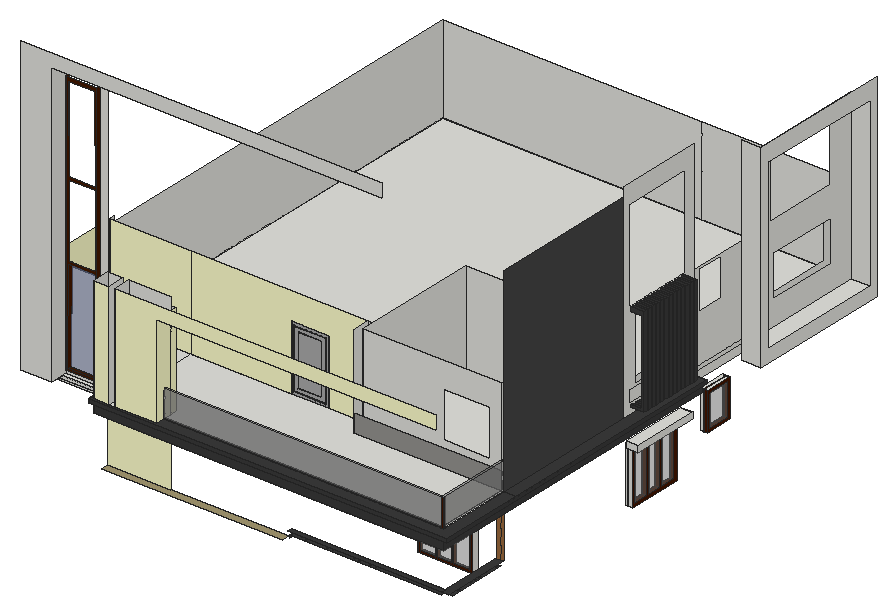
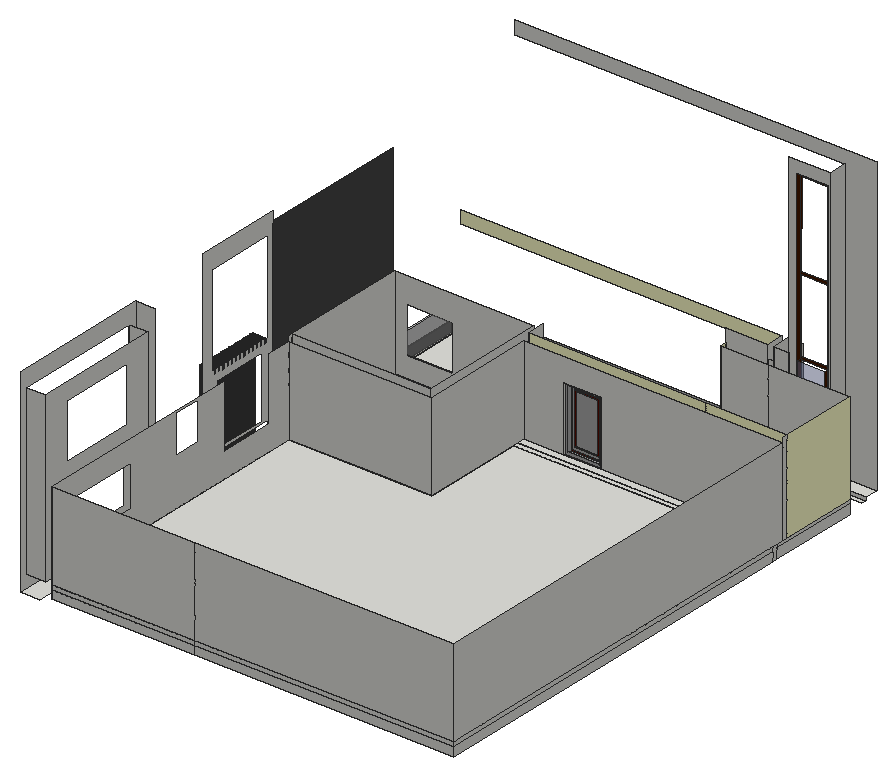
# SketchUp Ruby script. Lengths in inches.
U = 1.inch
M = Sketchup.active_model
def pt(a) = Geom::Point3d.new(a.map { |v| v * U })
def face(e, loops, mat)
  f = e.add_face(loops[0].map { |a| pt(a) })
  loops[1..].each { |l| e.add_face(l.map { |a| pt(a) }).erase! }
  f.material = f.back_material = mat if mat
  f
end
# faces: each face lists its corners as indices into pts; further lists are holes
def faces(e, pts, list, mat = nil) = list.each { |f| face(e, (f[0].is_a?(Array) ? f : [f]).map { |l| l.map { |i| pts[i] } }, mat) }
# xy, xz, yz: faces in a plane at the given z, y or x. An outline is a flat list of corners, or four numbers for a rectangle; further outlines are holes
def ring(l) = l.size == 4 ? [[l[0], l[1]], [l[2], l[1]], [l[2], l[3]], [l[0], l[3]]] : l.each_slice(2).to_a
def flat(e, list, mat, &to3) = list.each { |f| face(e, (f[0].is_a?(Array) ? f : [f]).map { |l| ring(l).map { |u, v| to3.(u, v) } }, mat) }
def xy(e, z, list, mat = nil) = flat(e, list, mat) { |x, y| [x, y, z] }
def xz(e, y, list, mat = nil) = flat(e, list, mat) { |x, z| [x, y, z] }
def yz(e, x, list, mat = nil) = flat(e, list, mat) { |y, z| [x, y, z] }
def lines(e, pts, list) = list.each { |a, b| e.add_line(pt(pts[a]), pt(pts[b])) }
# prism: a flat outline (further loops are holes) pulled along v
def prism(e, loops, v, mat = nil)
  f = face(e, loops, mat); d = Geom::Vector3d.new(v.map { |x| x * U })
  f.pushpull(f.normal.samedirection?(d) ? d.length : -d.length)
end
def box(e, o, s, mat = nil) = prism(e, [[o, [o[0] + s[0], o[1], o[2]], [o[0] + s[0], o[1] + s[1], o[2]], [o[0], o[1] + s[1], o[2]]]], [0, 0, s[2]], mat)
def at(x, y, z, deg = 0) = Geom::Transformation.translation(pt([x, y, z])) * Geom::Transformation.rotation(ORIGIN, Z_AXIS, deg.degrees)
def axes(o, x, y, z) = Geom::Transformation.new([*x, 0, *y, 0, *z, 0, *pt(o).to_a, 1])
def part(name) = M.definitions.add(name)
# library, detail: a bought-in or finely detailed component or shape, given as its bounding box
def library(name, o, s) = part(name).tap { |d| box(d.entities, o, s) }
def detail(e, o, s) = box(e.add_group.entities, o, s)
def put(e, d, t, mat = nil) = e.add_instance(d, t).tap { |i| i.material = mat if mat }
def group(e, t, mat = nil) = e.add_group.tap { |g| g.transformation = t; g.material = mat if mat }.entities
root = M.entities
M.materials.add("[Color A08]").color = [67, 22, 0]
M.materials.add("[Color A08]1").color = [91, 11, 0]
M.materials.add("[Color B08]").color = [69, 25, 0]
M.materials.add("[Color E01]").color = [255, 255, 204]
M.materials.add("[Color M03]").color = [170, 170, 170]
M.materials.add("[Color M07]").color = [58, 58, 58]
M.materials.add("[Granite Dark Gray]").color = [69, 68, 68]
M.materials.add("[Granite Light Gray]").color = [149, 148, 144]
M.materials.add("[Translucent Glass Gray]").color = [128, 128, 128]
M.materials["[Translucent Glass Gray]"].alpha = 0.5
M.materials.add("[Translucent Glass Sky Reflection]").color = [126, 138, 183]
M.materials["[Translucent Glass Sky Reflection]"].alpha = 0.52
M.materials.add("[Wood Floor]").color = [155, 105, 61]
M.materials.add("[Wood Lumber ButtJoined]").color = [164, 152, 112]
c1 = part("Group\#2")
xy(c1.entities,0,[[0,0,74.4375,5]],"[Color A08]")
xy(c1.entities,4.02,[[4.02,0,24.3,5],[27.19,0,45.86,5],[48.76,0,70.42,5]],"[Color A08]")
xy(c1.entities,85.67,[[4.02,0,24.3,5],[27.19,0,45.86,5],[48.76,0,70.42,5]],"[Color A08]")
xy(c1.entities,89.6875,[[0,0,74.4375,5]],"[Color A08]")
xz(c1.entities,0,[[[0,0,74.4375,89.6875],[48.76,4.02,70.42,85.67],[4.02,4.02,24.3,85.67],[27.19,4.02,45.86,85.67]]],"[Color A08]")
xz(c1.entities,0,[[4.02,4.02,24.3,85.67],[27.19,4.02,45.86,85.67],[48.76,4.02,70.42,85.67]],"[Translucent Glass Gray]")
xz(c1.entities,5,[[[0,0,74.4375,89.6875],[48.76,4.02,70.42,85.67],[4.02,4.02,24.3,85.67],[27.19,4.02,45.86,85.67]]],"[Color A08]")
yz(c1.entities,0,[[0,0,5,89.6875]],"[Color A08]")
yz(c1.entities,4.02,[[0,4.02,5,85.67]],"[Color A08]")
yz(c1.entities,24.3,[[0,4.02,5,85.67]],"[Color A08]")
yz(c1.entities,27.19,[[0,4.02,5,85.67]],"[Color A08]")
yz(c1.entities,45.86,[[0,4.02,5,85.67]],"[Color A08]")
yz(c1.entities,48.76,[[0,4.02,5,85.67]],"[Color A08]")
yz(c1.entities,70.42,[[0,4.02,5,85.67]],"[Color A08]")
yz(c1.entities,74.4375,[[0,0,5,89.6875]],"[Color A08]")
c2 = part("Group\#1")
xy(c2.entities,0,[[0,0,26.5,5]],"[Color A08]")
xy(c2.entities,2.85,[[2.85,0,23.65,5]],"[Color A08]")
xy(c2.entities,35.15,[[2.85,0,23.65,5]],"[Color A08]")
xy(c2.entities,38,[[0,0,26.5,5]],"[Color A08]")
xz(c2.entities,0,[[[0,0,26.5,38],[2.85,2.85,23.65,35.15]]],"[Color A08]")
xz(c2.entities,0,[[2.85,2.85,23.65,35.15]],"[Translucent Glass Gray]")
xz(c2.entities,5,[[[0,0,26.5,38],[2.85,2.85,23.65,35.15]]],"[Color A08]")
yz(c2.entities,0,[[0,0,5,38]],"[Color A08]")
yz(c2.entities,2.85,[[0,2.85,5,35.15]],"[Color A08]")
yz(c2.entities,23.65,[[0,2.85,5,35.15]],"[Color A08]")
yz(c2.entities,26.5,[[0,0,5,38]],"[Color A08]")
c3 = part("Group\#3")
xy(c3.entities,0,[[0,0,48,5]],"[Color M03]")
xy(c3.entities,2.98,[[2.98,0,45.02,5]],"[Color M03]")
xy(c3.entities,81.02,[[2.98,0,45.02,5]],"[Color M03]")
xy(c3.entities,84,[[0,0,48,5]],"[Color M03]")
xz(c3.entities,0,[[[2.98,2.98,45.02,81.02],[4.42,4.42,43.58,79.58]],[[8.55,8.55,39.45,75.45],[9.61,9.61,38.39,74.39]]],"[Color A08]1")
xz(c3.entities,0,[[[0,0,48,84],[2.98,2.98,45.02,81.02]],[[4.42,4.42,43.58,79.58],[8.55,8.55,39.45,75.45]],[9.61,9.61,38.39,74.39]],"[Color M03]")
xz(c3.entities,5,[[[0,0,48,84],[2.98,2.98,45.02,81.02]]],"[Color M03]")
yz(c3.entities,0,[[0,0,5,84]],"[Color M03]")
yz(c3.entities,2.98,[[0,2.98,5,81.02]],"[Color M03]")
yz(c3.entities,45.02,[[0,2.98,5,81.02]],"[Color M03]")
yz(c3.entities,48,[[0,0,5,84]],"[Color M03]")
xy(root,166.03,[[531,322.23,540,393.92]])
xy(root,166.65,[[427.93,113.4375,499.81,121.0625]])
xy(root,188.5625,[[94.8,18,330.17,27]],"[Wood Lumber ButtJoined]")
xy(root,191.28,[[533.85,35.98,537.54,37.92]])
xy(root,191.34,[[533.85,49.61,537.54,51.55],[533.85,97.3,537.54,99.23]])
xy(root,191.35,[[[531,31.22,540,109.22],[533.85,90.48,537.54,92.42],[533.85,83.67,537.54,85.61],[533.85,56.42,537.54,58.36]]],"[Color M07]")
xy(root,191.4,[[533.85,42.8,537.54,44.73]])
xy(root,191.47,[[533.85,70.05,537.54,71.98]])
xy(root,191.53,[[533.85,63.23,537.54,65.17],[533.85,76.86,537.54,78.8]])
xy(root,191.78,[[533.85,104.11,537.54,106.05]])
xy(root,192.09,[[344.98,26.53,346.42,29.97]])
xy(root,192.28,[[372.98,26.53,374.42,29.97],[455.98,26.53,457.42,29.97]])
xy(root,192.34,[[365.98,26.53,367.42,29.97],[468.98,26.53,470.42,29.97],[481.98,26.53,483.42,29.97],[501.48,26.53,502.92,29.97]])
xy(root,192.35,[[[333.39,24.875,531,31.22],[337.98,26.53,339.42,29.97],[358.98,26.53,360.42,29.97],[400.98,26.53,402.42,29.97],[393.98,26.53,395.42,29.97],[407.98,26.53,409.42,29.97],[428.98,26.53,430.42,29.97],[449.48,26.53,450.92,29.97],[475.48,26.53,476.92,29.97],[514.3,26.53,515.73,29.97],[507.98,26.53,509.42,29.97],[494.98,26.53,496.42,29.97],[488.48,26.53,489.92,29.97]]],"[Color M07]")
xy(root,192.4,[[351.98,26.53,353.42,29.97],[435.98,26.53,437.42,29.97]])
xy(root,192.65,[[379.98,26.53,381.42,29.97]])
xy(root,193.03,[[421.98,26.53,423.42,29.97]])
xy(root,193.16,[[386.98,26.53,388.42,29.97]])
xy(root,193.4,[[414.98,26.53,416.42,29.97]])
xy(root,193.47,[[442.98,26.53,444.42,29.97]])
xy(root,194.84,[[462.48,26.53,463.92,29.97]])
xy(root,195.5625,[[[330.17,24.875,531,31.22],[522.48,26.53,523.92,29.97]],[531,24.875,540,113.4375],[522.48,26.53,523.92,29.97]],"[Color M07]")
xy(root,199.38,[[531,443.95,540,480.39]])
xy(root,224.19,[[246.2,154.125,294.2,161.0625]])
xy(root,232.9,[[427.93,113.4375,499.81,121.0625]])
xy(root,237.71,[[531,322.23,540,393.92]])
xy(root,239.1,[[540,313.39,554.5,401.58]])
xy(root,247.29,[[540,313.39,554.5,401.58]])
xy(root,248.63,[[531,443.95,540,480.39]])
xy(root,259.5625,[[540,499.48,564.9375,687]])
xy(root,259.5625,[[94.8,3.875,176.76,27]],"[Color M07]")
xy(root,259.5625,[[176.76,3.875,176.76,36,9,36,9,154.125,345.1875,154.125,345.1875,113.4375,540,113.4375,540,421.98,549.8125,421.98,549.8125,3.875]],"[Wood Floor]")
xy(root,270.5625,[[9,161.0625,9,678,531,678,531,294,345.1875,294,345.1875,161.0625]])
xy(root,272.125,[[176.76,3.875,549.8125,3.875,549.8125,421.98,540,421.98,540,113.4375,345.1875,113.4375,345.1875,154.125,9,154.125,9,36,176.76,36]])
xy(root,272.125,[[91.49,0,556.4375,3.875],[549.8125,3.875,556.4375,421.98]],"[Color M07]")
xy(root,272.3125,[[0,21.625,94.8,27]])
xy(root,276.5625,[[0,3.875,40.88,21.625],[94.8,3.875,114.93,27],[114.93,3.875,122.06,27],[122.06,3.875,176.76,27],[176.76,15.4375,176.76,17.37,537.49,17.37,537.49,113.4375,540,113.4375,540,15.4375],
  [176.76,17.37,537.49,17.37,537.49,113.4375,345.1875,113.4375,345.1875,137.125,293.49,137.125,293.49,144.4375,245.49,144.4375,245.49,137.125,114.93,137.125,114.93,36,176.76,36],[40.88,21.625,94.8,27],[9,36,114.93,137.125],[351.1875,121.0625,531,288],[9,137.125,245.49,144.4375],
  [293.49,137.125,345.1875,144.4375],[9,144.4375,345.1875,154.125],[9,154.125,345.1875,161.0625],[9,161.0625,345.1875,161.0625,345.1875,294,531,294,531,678,9,678],[540,510.97,564.9375,677.39]])
xy(root,276.5625,[[91.49,0,556.4375,0,556.4375,113.4375,540,113.4375,540,15.4375,176.76,15.4375,176.76,3.875,91.49,3.875],[91.49,3.875,94.8,21.625],[540,113.4375,556.4375,421.98]],"[Color M07]")
xy(root,283.84,[[44.88,22.1875,85.01,27]],"[Color B08]")
xy(root,284.79,[[540,393.85,558.125,397.23],[540.07,400.66,558.125,404.04]],"[Color M07]")
xy(root,284.88,[[540,318.91,558.125,322.29],[540,325.73,558.125,329.1],[540,332.54,558.125,335.91],[540,339.35,558.125,342.73],[540,346.16,558.125,349.54],
  [540,352.98,558.125,356.35],[540,359.79,558.125,363.16],[540,366.6,558.125,369.98],[540,373.41,558.125,376.79],[540,380.23,558.125,383.6],
  [540,387.04,558.125,390.41]],"[Color M07]")
xy(root,286.45,[[47.49,22.1875,82.4,27]],"[Color B08]")
xz(root,0,[[91.49,272.125,556.4375,276.5625]],"[Color M07]")
xz(root,3.875,[[0,276.5625,40.88,276.5625,40.88,641.625,469.36,641.625,469.36,658.875,0,658.875]])
xz(root,3.875,[[94.8,276.5625,114.93,413.5625],[122.06,276.5625,176.76,276.5625,176.76,396.5625,540,396.5625,540,413.5625,122.06,413.5625]],"[Color E01]")
xz(root,3.875,[[94.8,259.5625,549.8125,272.125]],"[Color M07]")
xz(root,15.4375,[[537.49,276.5625,540,312.5625]],"[Color A08]")
xz(root,15.4375,[[176.76,276.5625,537.49,312.5625]],"[Translucent Glass Gray]")
xz(root,17.37,[[176.76,276.5625,537.49,312.5625]],"[Translucent Glass Gray]")
xz(root,21.625,[[0,272.3125,91.49,276.5625]])
xz(root,22.1875,[[[44.88,283.84,85.01,626.03],[47.49,286.45,47.93,408.17,82.84,408.17,82.4,286.45],[48.29,509.67,47.49,607.67,47.49,621.29,82.4,621.29,82.4,607.67,83.2,509.67],[47.94,411.11,48.29,506.73,83.2,506.73,82.85,411.11]]],"[Color B08]")
xz(root,27,[[[40.88,276.5625,94.8,641.625],[44.88,283.84,85.01,626.03]],[94.8,276.5625,114.93,413.5625],[114.93,276.5625,122.06,396.5625],[122.06,276.5625,176.76,276.5625,176.76,396.5625,176.66,396.5625,176.66,413.5625,122.06,413.5625]])
xz(root,27,[[94.8,188.5625,176.76,259.5625]],"[Color E01]")
xz(root,27,[[47.49,286.45,82.4,286.45,82.84,408.17,47.93,408.17]],"[Translucent Glass Sky Reflection]")
xz(root,36,[[9,259.5625,176.76,272.125],[9,276.5625,114.93,396.5625],[114.93,276.5625,176.76,396.5625]])
xz(root,113.4375,[[345.1875,259.5625,351.24,272.125],[351.24,259.5625,356.12,272.125],[356.12,259.5625,360.99,272.125],[360.99,259.5625,365.87,272.125],[365.87,259.5625,370.74,272.125],
  [370.74,259.5625,375.62,272.125],[375.62,259.5625,380.49,272.125],[380.49,259.5625,385.37,272.125],[385.37,259.5625,390.24,272.125],[390.24,259.5625,395.12,272.125],
  [395.12,259.5625,399.99,272.125],[399.99,259.5625,404.87,272.125],[404.87,259.5625,409.74,272.125],[409.74,259.5625,414.62,272.125],[414.62,259.5625,419.49,272.125],
  [419.49,259.5625,424.37,272.125],[424.37,259.5625,429.24,272.125],[429.24,259.5625,434.12,272.125],[434.12,259.5625,438.99,272.125],[438.99,259.5625,443.87,272.125],
  [443.87,259.5625,448.74,272.125],[448.74,259.5625,453.62,272.125],[453.62,259.5625,458.49,272.125],[458.49,259.5625,463.37,272.125],[463.37,259.5625,468.24,272.125],
  [468.24,259.5625,473.12,272.125],[473.12,259.5625,477.99,272.125],[477.99,259.5625,482.87,272.125],[482.87,259.5625,487.74,272.125],[487.74,259.5625,492.62,272.125],
  [492.62,259.5625,497.49,272.125],[497.49,259.5625,502.37,272.125],[502.37,259.5625,507.24,272.125],[507.24,259.5625,512.12,272.125],[512.12,259.5625,516.99,272.125],
  [516.99,259.5625,521.87,272.125],[521.87,259.5625,526.74,272.125],[526.74,259.5625,531.62,272.125],[531.62,259.5625,536.49,272.125],[536.49,259.5625,540,272.125],
  [537.49,276.5625,540,312.5625]])
xz(root,113.4375,[[345.1875,276.5625,537.49,299.25]],"[Granite Light Gray]")
xz(root,113.4375,[[531.62,195.5625,536.49,259.5625],[536.49,195.5625,540,259.5625],[429.24,232.9,434.12,259.5625],[434.12,232.9,438.99,259.5625],[438.99,232.9,443.87,259.5625],
  [443.87,232.9,448.74,259.5625],[448.74,232.9,453.62,259.5625],[453.62,232.9,458.49,259.5625],[458.49,232.9,463.37,259.5625],[463.37,232.9,468.24,259.5625],
  [468.24,232.9,473.12,259.5625],[473.12,232.9,477.99,259.5625],[477.99,232.9,482.87,259.5625],[482.87,232.9,487.74,259.5625],[487.74,232.9,492.62,259.5625],
  [492.62,232.9,497.49,259.5625]],"[Wood Floor]")
xz(root,121.0625,[[351.1875,259.5625,531,276.5625],[[351.1875,276.5625,531,396.5625],[456,303.1875,516,363.1875]]])
xz(root,137.125,[[9,276.5625,114.93,396.5625],[114.93,276.5625,245.49,276.5625,245.49,360.5625,293.49,360.5625,293.49,276.5625,345.1875,276.5625,345.1875,396.5625,114.93,396.5625]],"[Color E01]")
xz(root,144.4375,[[9,276.5625,9,390.5625,345.1875,390.5625,345.1875,276.5625,293.49,276.5625,293.49,360.5625,245.49,360.5625,245.49,276.5625]])
xz(root,154.125,[[9,259.5625,345.1875,272.125],[9,272.125,345.1875,276.5625]])
xz(root,161.0625,[[9,259.5625,345.1875,270.5625],[9,270.5625,345.1875,276.5625]])
xz(root,288,[[351.1875,259.5625,531,276.5625],[351.1875,276.5625,531,396.5625]])
xz(root,294,[[345.1875,259.5625,531,270.5625],[345.1875,270.5625,387.03,276.5625],[387.03,270.5625,399.72,276.5625],[399.72,270.5625,531,276.5625],[345.1875,276.5625,531,390.5625]])
xz(root,313.39,[[540,239.1,554.5,247.29]])
xz(root,318.91,[[540,284.88,558.125,284.88,558.125,401.88,540,401.88,540,395.82,555.51,395.82,555.51,287.86,540,287.86]],"[Color M07]")
xz(root,322.23,[[531,166.03,540,237.71]])
xz(root,322.29,[[540,284.88,540,287.86,555.51,287.86,555.51,395.82,540,395.82,540,401.88,558.125,401.88,558.125,284.88]],"[Color M07]")
xz(root,325.73,[[540,284.88,558.125,284.88,558.125,401.88,540,401.88,540,395.82,555.51,395.82,555.51,287.86,540,287.86]],"[Color M07]")
xz(root,329.1,[[540,284.88,540,287.86,555.51,287.86,555.51,395.82,540,395.82,540,401.88,558.125,401.88,558.125,284.88]],"[Color M07]")
xz(root,332.54,[[540,284.88,558.125,284.88,558.125,401.88,540,401.88,540,395.82,555.51,395.82,555.51,287.86,540,287.86]],"[Color M07]")
xz(root,335.91,[[540,284.88,540,287.86,555.51,287.86,555.51,395.82,540,395.82,540,401.88,558.125,401.88,558.125,284.88]],"[Color M07]")
xz(root,339.35,[[540,284.88,558.125,284.88,558.125,401.88,540,401.88,540,395.82,555.51,395.82,555.51,287.86,540,287.86]],"[Color M07]")
xz(root,342.73,[[540,284.88,540,287.86,555.51,287.86,555.51,395.82,540,395.82,540,401.88,558.125,401.88,558.125,284.88]],"[Color M07]")
xz(root,346.16,[[540,284.88,558.125,284.88,558.125,401.88,540,401.88,540,395.82,555.51,395.82,555.51,287.86,540,287.86]],"[Color M07]")
xz(root,349.54,[[540,284.88,540,287.86,555.51,287.86,555.51,395.82,540,395.82,540,401.88,558.125,401.88,558.125,284.88]],"[Color M07]")
xz(root,352.98,[[540,284.88,558.125,284.88,558.125,401.88,540,401.88,540,395.82,555.51,395.82,555.51,287.86,540,287.86]],"[Color M07]")
xz(root,356.35,[[540,284.88,540,287.86,555.51,287.86,555.51,395.82,540,395.82,540,401.88,558.125,401.88,558.125,284.88]],"[Color M07]")
xz(root,359.79,[[540,284.88,558.125,284.88,558.125,401.88,540,401.88,540,395.82,555.51,395.82,555.51,287.86,540,287.86]],"[Color M07]")
xz(root,363.16,[[540,284.88,540,287.86,555.51,287.86,555.51,395.82,540,395.82,540,401.88,558.125,401.88,558.125,284.88]],"[Color M07]")
xz(root,366.6,[[540,284.88,558.125,284.88,558.125,401.88,540,401.88,540,395.82,555.51,395.82,555.51,287.86,540,287.86]],"[Color M07]")
xz(root,369.98,[[540,284.88,540,287.86,555.51,287.86,555.51,395.82,540,395.82,540,401.88,558.125,401.88,558.125,284.88]],"[Color M07]")
xz(root,373.41,[[540,284.88,558.125,284.88,558.125,401.88,540,401.88,540,395.82,555.51,395.82,555.51,287.86,540,287.86]],"[Color M07]")
xz(root,376.79,[[540,284.88,540,287.86,555.51,287.86,555.51,395.82,540,395.82,540,401.88,558.125,401.88,558.125,284.88]],"[Color M07]")
xz(root,380.23,[[540,284.88,558.125,284.88,558.125,401.88,540,401.88,540,395.82,555.51,395.82,555.51,287.86,540,287.86]],"[Color M07]")
xz(root,383.6,[[540,284.88,540,287.86,555.51,287.86,555.51,395.82,540,395.82,540,401.88,558.125,401.88,558.125,284.88]],"[Color M07]")
xz(root,387.04,[[540,284.88,558.125,284.88,558.125,401.88,540,401.88,540,395.82,555.51,395.82,555.51,287.86,540,287.86]],"[Color M07]")
xz(root,390.41,[[540,284.88,540,287.86,555.51,287.86,555.51,395.82,540,395.82,540,401.88,558.125,401.88,558.125,284.88]],"[Color M07]")
xz(root,393.85,[[540,284.79,558.125,284.79,558.125,401.88,540,401.88,540,395.82,555.51,395.82,555.51,287.86,540,287.86]],"[Color M07]")
xz(root,393.92,[[531,166.03,540,237.71]])
xz(root,397.23,[[540,284.79,540,287.86,555.51,287.86,555.51,395.82,540,395.82,540,401.88,558.125,401.88,558.125,284.79]],"[Color M07]")
xz(root,400.66,[[540.07,284.79,558.125,284.79,558.125,401.88,540,401.88,540,395.82,555.51,395.82,555.51,287.86,540.07,287.86]],"[Color M07]")
xz(root,401.58,[[540,239.1,554.5,247.29]])
xz(root,404.04,[[540.07,284.79,540.07,287.86,555.51,287.86,555.51,395.82,540,395.82,540,401.88,558.125,401.88,558.125,284.79]],"[Color M07]")
xz(root,421.98,[[540,259.5625,549.8125,272.125],[540,272.125,556.4375,276.5625]],"[Color M07]")
xz(root,443.95,[[531,199.38,540,248.63]])
xz(root,480.39,[[531,199.38,540,248.63]])
xz(root,499.48,[[540,259.5625,564.9375,515.86]])
xz(root,510.97,[[540,276.5625,564.9375,493.64]])
xz(root,677.39,[[540,276.5625,564.9375,493.64]])
xz(root,678,[[9,259.5625,345.75,270.5625],[345.75,259.5625,531,270.5625],[9,270.5625,345.75,276.5625],[345.75,270.5625,531,276.5625],[9,276.5625,345.75,390.5625],
  [345.75,276.5625,531,390.5625]])
yz(root,9,[[36,259.5625,154.125,272.125],[154.125,259.5625,161.0625,276.5625],[161.0625,259.5625,678,270.5625],[161.0625,270.5625,678,276.5625],[36,272.125,154.125,276.5625],
  [137.125,276.5625,144.4375,396.5625],[144.4375,276.5625,678,390.5625]])
yz(root,9,[[36,276.5625,137.125,396.5625]],"[Color E01]")
yz(root,40.88,[[3.875,276.5625,27,641.625]])
yz(root,44.88,[[22.1875,283.84,27,626.03]],"[Color B08]")
yz(root,85.01,[[22.1875,283.84,27,626.03]],"[Color B08]")
yz(root,91.49,[[0,272.125,0,276.5625,21.625,276.5625,21.625,272.3125,3.875,272.125]],"[Color M07]")
yz(root,94.8,[[3.875,276.5625,27,413.5625]])
yz(root,94.8,[[3.875,259.5625,3.875,272.125,21.625,272.3125,27,272.3125,27,259.5625]],"[Color M07]")
yz(root,114.93,[[3.875,276.5625,27,413.5625]])
yz(root,122.06,[[3.875,276.5625,27,413.5625]])
yz(root,176.76,[[27,259.5625,36,272.125],[15.4375,276.5625,17.37,312.5625]])
yz(root,176.76,[[3.875,276.5625,15.4375,276.5625,15.4375,315.5625,17.37,315.5625,17.37,276.5625,27,276.5625,27,396.5625,3.875,396.5625],[27,276.5625,36,396.5625]],"[Color E01]")
yz(root,245.49,[[137.125,276.5625,144.4375,360.5625]])
yz(root,293.49,[[137.125,276.5625,144.4375,360.5625]])
yz(root,333.39,[[24.875,188.5625,31.22,192.35]],"[Color M07]")
yz(root,345.1875,[[113.4375,259.5625,154.125,272.125],[161.0625,259.5625,294,270.5625],[161.0625,270.5625,294,276.5625],[113.4375,276.5625,137.125,396.5625],[144.4375,276.5625,294,390.5625]])
yz(root,351.1875,[[121.0625,259.5625,288,276.5625],[121.0625,276.5625,288,396.5625]])
yz(root,427.93,[[113.4375,166.65,121.0625,232.9]])
yz(root,499.81,[[113.4375,166.65,121.0625,232.9]])
yz(root,531,[[121.0625,259.5625,288,276.5625],[288,259.5625,294,276.5625],[294,259.5625,678,270.5625],[294,270.5625,678,276.5625],[121.0625,276.5625,288,396.5625],
  [288,276.5625,294,396.5625],[[294,276.5625,294,390.5625,326.1,390.5625,326.1,308.5625,399.73,308.5625,399.73,390.5625,678,390.5625,678,276.5625],[550.29,308.49,644.04,362.37],[441.39,338.69,477.83,387.94]]])
yz(root,537.49,[[17.37,276.5625,113.4375,312.5625]],"[Translucent Glass Gray]")
yz(root,540,[[113.4375,259.5625,117.98,272.125],[117.98,259.5625,122.98,272.125],[122.98,259.5625,127.98,272.125],[127.98,259.5625,132.98,272.125],[132.98,259.5625,137.98,272.125],
  [137.98,259.5625,142.98,272.125],[142.98,259.5625,147.98,272.125],[147.98,259.5625,152.98,272.125],[152.98,259.5625,157.98,272.125],[157.98,259.5625,162.98,272.125],
  [162.98,259.5625,167.98,272.125],[167.98,259.5625,172.98,272.125],[172.98,259.5625,177.98,272.125],[177.98,259.5625,182.98,272.125],[182.98,259.5625,187.98,272.125],
  [187.98,259.5625,192.98,272.125],[192.98,259.5625,197.98,272.125],[197.98,259.5625,202.98,272.125],[202.98,259.5625,207.98,272.125],[207.98,259.5625,212.98,272.125],
  [212.98,259.5625,217.98,272.125],[217.98,259.5625,222.98,272.125],[222.98,259.5625,227.98,272.125],[227.98,259.5625,232.98,272.125],[232.98,259.5625,237.98,272.125],
  [237.98,259.5625,242.98,272.125],[242.98,259.5625,247.98,272.125],[247.98,259.5625,252.98,272.125],[252.98,259.5625,257.98,272.125],[257.98,259.5625,262.98,272.125],
  [262.98,259.5625,267.98,272.125],[267.98,259.5625,272.98,272.125],[272.98,259.5625,277.98,272.125],[277.98,259.5625,282.98,272.125],[282.98,259.5625,287.98,272.125],
  [287.98,259.5625,292.98,272.125],[292.98,259.5625,421.98,272.125],[[308.13,276.5625,421.98,545.5625],[318.91,395.82,318.91,401.88,316.14,401.88,316.14,521.1,408.01,521.1,408.01,401.88,404.04,401.88,404.04,395.82,400.66,395.82,400.66,401.88,397.23,401.88,397.23,395.82,393.85,395.82,393.85,401.88,390.41,401.88,390.41,395.82,387.04,395.82,387.04,401.88,383.6,401.88,383.6,395.82,380.23,395.82,380.23,401.88,376.79,401.88,376.79,395.82,373.41,395.82,373.41,401.88,369.98,401.88,369.98,395.82,366.6,395.82,366.6,401.88,363.16,401.88,363.16,395.82,359.79,395.82,359.79,401.88,356.35,401.88,356.35,395.82,352.98,395.82,352.98,401.88,349.54,401.88,349.54,395.82,346.16,395.82,346.16,401.88,342.73,401.88,342.73,395.82,339.35,395.82,339.35,401.88,335.91,401.88,335.91,395.82,332.54,395.82,332.54,401.88,329.1,401.88,329.1,395.82,325.73,395.82,325.73,401.88,322.29,401.88,322.29,395.82],[326.1,308.5625,399.73,388.5],[316.71,288.91,407.9,305.97],[393.85,284.79,397.23,287.86],[318.91,284.88,322.29,287.86],[325.73,284.88,329.1,287.86],[332.54,284.88,335.91,287.86],[339.35,284.88,342.73,287.86],[346.16,284.88,349.54,287.86],[352.98,284.88,356.35,287.86],[359.79,284.88,363.16,287.86],[366.6,284.88,369.98,287.86],[373.41,284.88,376.79,287.86],[380.23,284.88,383.6,287.86],[387.04,284.88,390.41,287.86]],[[510.97,276.5625,677.39,493.64],[545.63,400.9,643.13,472.21],[550.29,308.49,644.04,362.37]]])
yz(root,540,[[15.4375,276.5625,17.37,312.5625]],"[Color A08]")
yz(root,540,[[113.4375,276.5625,308.13,533.5625]],"[Granite Dark Gray]")
yz(root,540,[[17.37,276.5625,113.4375,312.5625]],"[Translucent Glass Gray]")
yz(root,540.07,[[400.66,284.79,404.04,287.86]])
yz(root,549.8125,[[3.875,259.5625,421.98,272.125]],"[Color M07]")
yz(root,554.5,[[313.39,239.1,401.58,247.29]])
yz(root,556.4375,[[0,272.125,421.98,276.5625]],"[Color M07]")
yz(root,558.125,[[393.85,284.79,397.23,401.88],[400.66,284.79,404.04,401.88],[318.91,284.88,322.29,401.88],[325.73,284.88,329.1,401.88],[332.54,284.88,335.91,401.88],
  [339.35,284.88,342.73,401.88],[346.16,284.88,349.54,401.88],[352.98,284.88,356.35,401.88],[359.79,284.88,363.16,401.88],[366.6,284.88,369.98,401.88],
  [373.41,284.88,376.79,401.88],[380.23,284.88,383.6,401.88],[387.04,284.88,390.41,401.88]],"[Color M07]")
yz(root,564.9375,[[[499.48,259.5625,687,515.86],[510.97,276.5625,677.39,493.64]]])
p = [[94.8,21.625,272.3125],[94.8,3.875,272.125],[91.49,3.875,272.125],[91.49,21.625,272.3125],[47.49,27,286.45],[47.93,27,408.17],
  [47.93,22.1875,408.17],[47.49,22.1875,286.45],[82.84,27,408.17],[82.4,27,286.45],[82.4,22.1875,286.45],[82.84,22.1875,408.17]]
faces(root,p,[[0,1,2,3]],"[Color M07]")
faces(root,p,[[4,5,6,7],[8,9,10,11]],"[Color B08]")
put(root,c1,axes([540,322.43,166.03],[0,0.96031,0],[-1.23966,0,0],[0,0,0.79476]))
put(root,c1,axes([183.26,261.3,166.03],[0,0.96031,0],[-1.23966,0,0],[0,0,0.79476]))
put(root,c1,axes([427.93,113.4375,166.65],[0.96558,0,0],[0,0.5952,0],[0,0,0.73868]))
put(root,c2,axes([540,443.95,199.38],[0,1.375,0],[-1,0,0],[0,0,1.29605]))
put(root,c3,at(245.49,137.125,276.5625))
